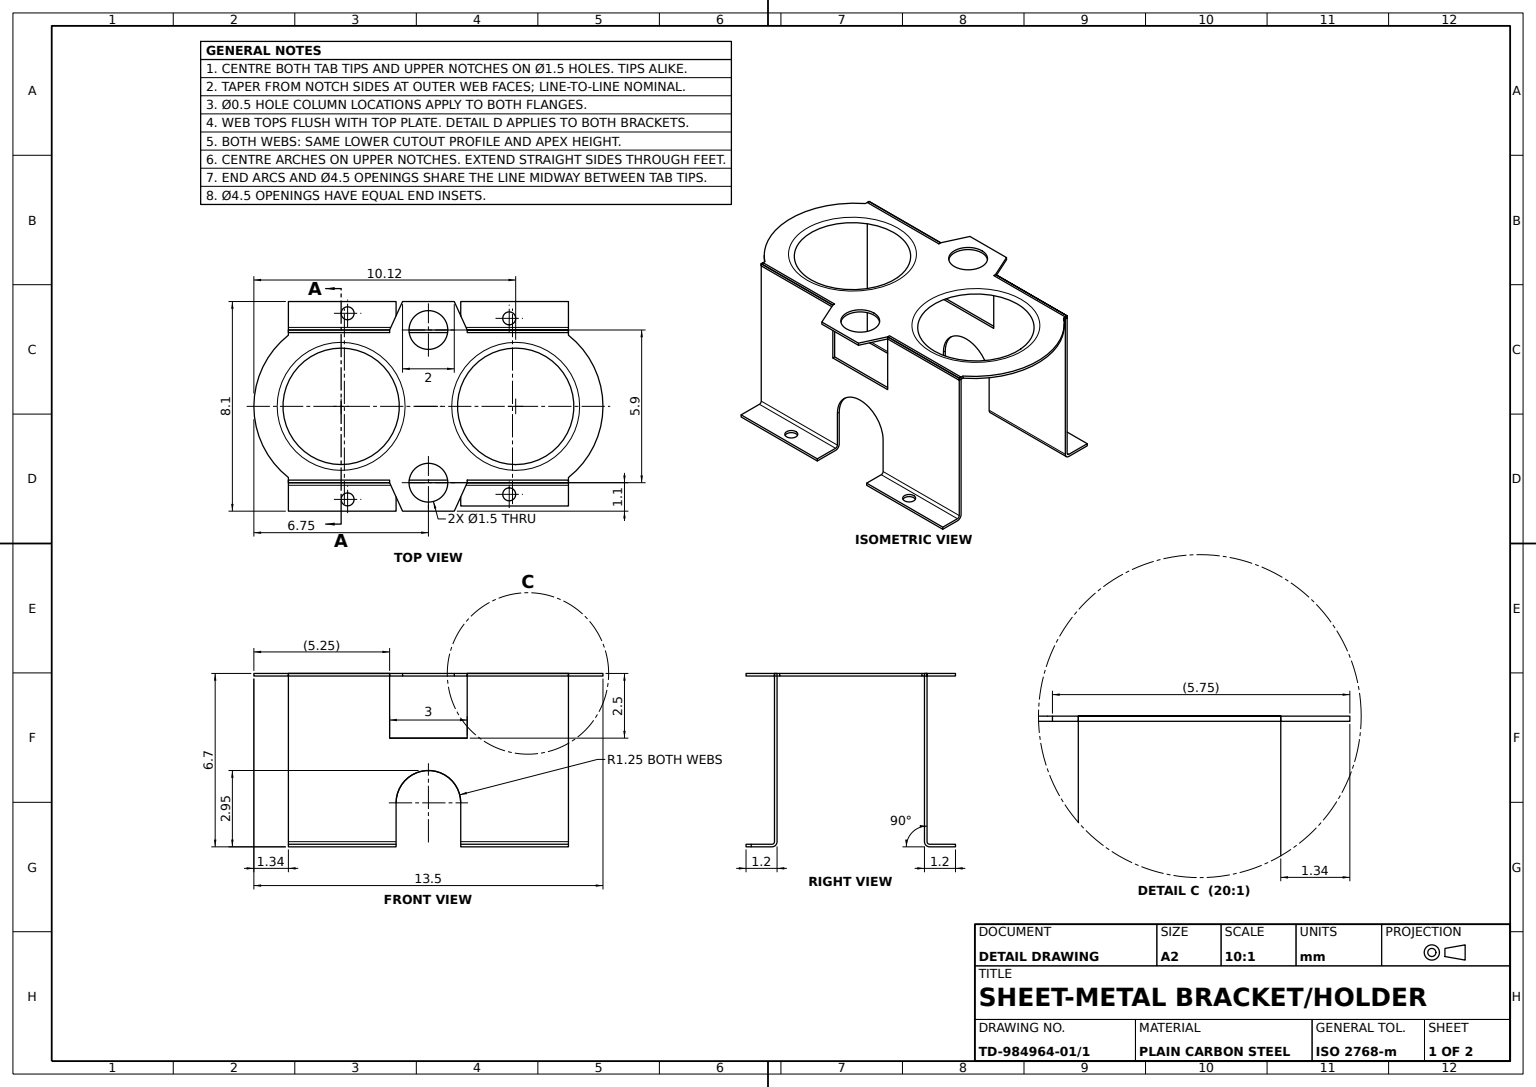
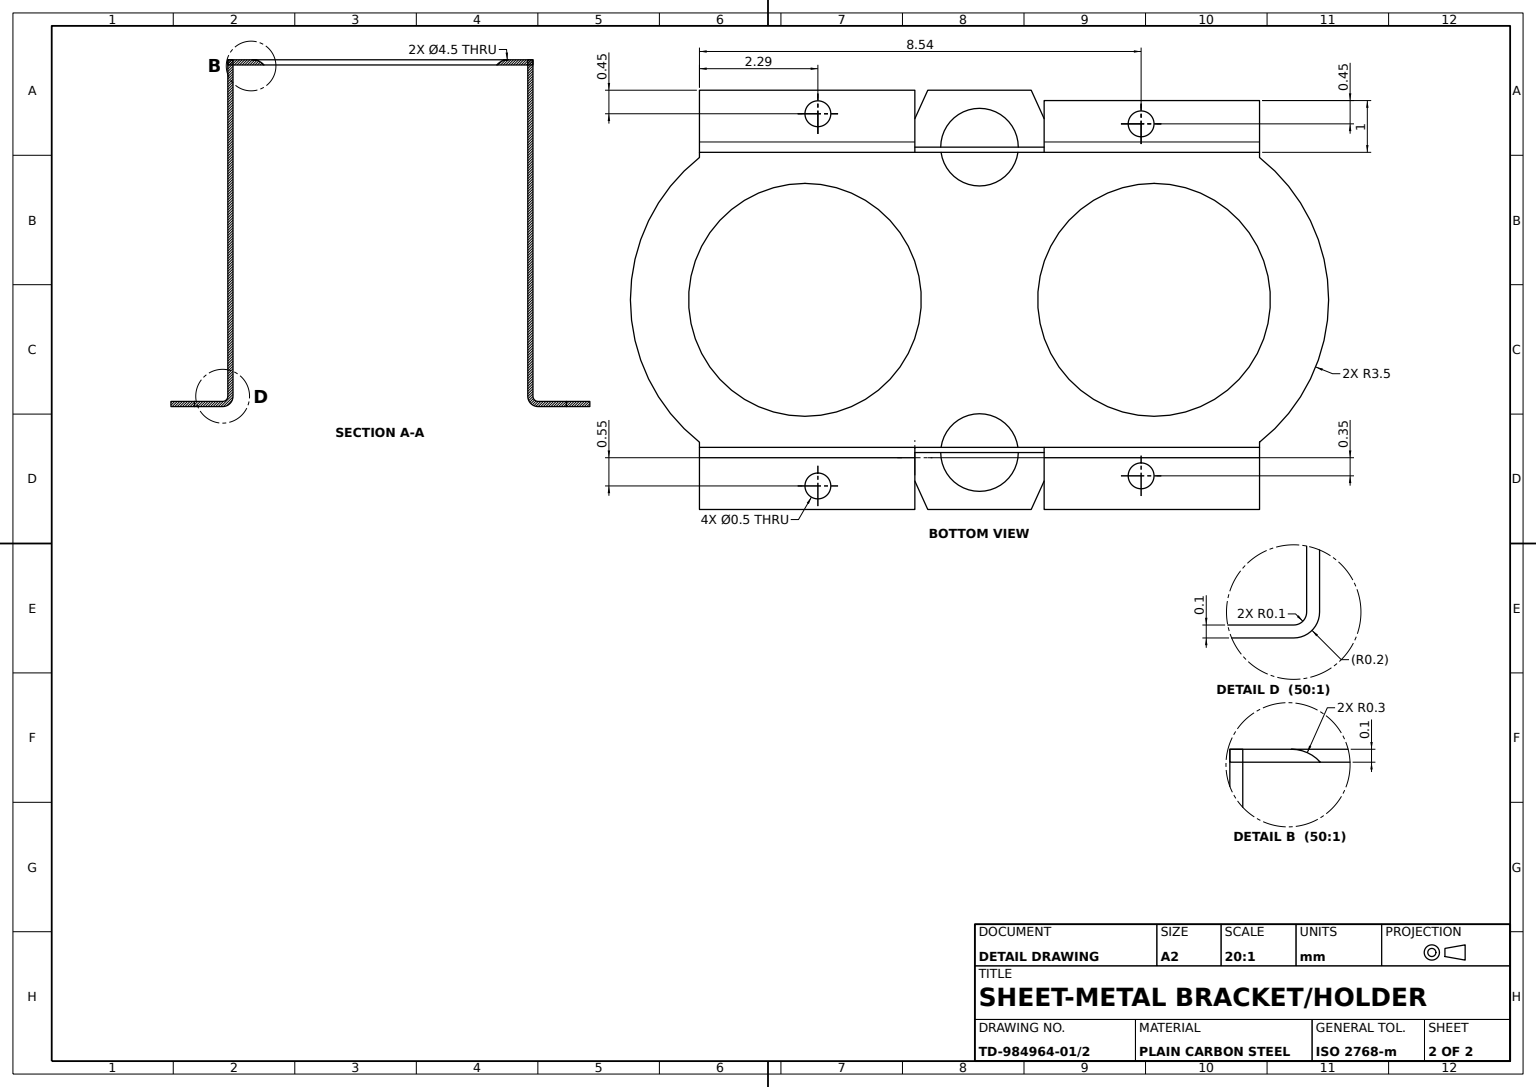
solid
v1 (3.375,0,-2.473607)
v2 (3.375,0,2.473607)
e1 v1 v2 CIRCLE(AX(P(3.375,0,0),D(0,-1,0),D(0,0,1)),2.473607)
v3 (3.375,-0.1,-2.25)
e2 v1 v3 CIRCLE(AX(P(3.375,-0.3,-2.473607),D(1,0,0),D(0,0,-1)),0.3)
v4 (3.375,-0.1,2.25)
e3 v4 v3 CIRCLE(AX(P(3.375,-0.1,0),D(0,1,0),D(0,0,-1)),2.25)
e4 v2 v4 CIRCLE(AX(P(3.375,-0.3,2.473607),D(-1,0,0),D(0,0,1)),0.3)
face TORUS(AX(P(3.375,-0.3,0),D(0,1,0),D(0,0,1)),2.473607,0.3) [-e1 e2 -e3 -e4]
v5 (-5.414993,0,-2.95)
v6 (-5.414993,0,-2.75)
e5 v5 v6 LINE
v7 (-5.414993,-0.1,-2.95)
e6 v7 v5 LINE
v8 (-5.414993,-0.1,-2.75)
e7 v7 v8 LINE
e8 v8 v6 LINE
face PLANE(AX(P(-5.414993,-0.1,-2.95),D(-1,0,0),D(0,0,1))) [-e5 -e6 e7 e8]
v9 (-1,0,4.05)
v10 (1,0,4.05)
e9 v9 v10 LINE
v11 (-1,-0.1,4.05)
e10 v11 v9 LINE
v12 (1,-0.1,4.05)
e11 v11 v12 LINE
e12 v12 v10 LINE
face PLANE(AX(P(-1,-0.1,4.05),D(0,0,1),D(1,0,0))) [-e9 -e10 e11 e12]
v13 (-1.5,-0.1,-2.95)
e13 v13 v7 LINE
v14 (-1.5,0,-2.95)
e14 v14 v5 LINE
e15 v13 v14 LINE
face PLANE(AX(P(-5.414993,-0.1,-2.95),D(0,0,-1),D(-1,0,0))) [e13 e6 -e14 -e15]
v15 (-1,-0.1,-4.05)
v16 (-1,0,-4.05)
e16 v15 v16 LINE
e17 v15 v13 LINE
e18 v16 v14 LINE
face PLANE(AX(P(-1,-0.1,-4.05),D(-0.910366477,0,-0.413802944),D(-0.413802944,0,0.910366477))) [-e16 e17 e15 -e18]
v17 (1.5,-0.1,2.95)
e19 v12 v17 LINE
v18 (1.5,0,2.95)
e20 v17 v18 LINE
e21 v10 v18 LINE
face PLANE(AX(P(1,-0.1,4.05),D(0.910366477,0,0.413802944),D(0.413802944,0,-0.910366477))) [-e12 e19 e20 -e21]
v19 (-3.375,0,2.473607)
v20 (-3.375,0,-2.473607)
e22 v19 v20 CIRCLE(AX(P(-3.375,0,0),D(0,-1,0),D(0,0,1)),2.473607)
v21 (-3.375,-0.1,2.25)
e23 v19 v21 CIRCLE(AX(P(-3.375,-0.3,2.473607),D(-1,0,0),D(0,0,1)),0.3)
v22 (-3.375,-0.1,-2.25)
e24 v22 v21 CIRCLE(AX(P(-3.375,-0.1,0),D(0,1,0),D(0,0,1)),2.25)
e25 v20 v22 CIRCLE(AX(P(-3.375,-0.3,-2.473607),D(1,0,0),D(0,0,-1)),0.3)
face TORUS(AX(P(-3.375,-0.3,0),D(0,1,0),D(0,0,1)),2.473607,0.3) [-e22 e23 -e24 -e25]
v23 (5.414993,0,2.95)
v24 (5.414993,0,2.75)
e26 v23 v24 LINE
v25 (5.414993,-0.1,2.95)
e27 v25 v23 LINE
v26 (5.414993,-0.1,2.75)
e28 v25 v26 LINE
e29 v26 v24 LINE
face PLANE(AX(P(5.414993,-0.1,2.95),D(1,0,0),D(0,0,-1))) [-e26 -e27 e28 e29]
e30 v17 v25 LINE
e31 v18 v23 LINE
face PLANE(AX(P(1.5,-0.1,2.95),D(0,0,1),D(1,0,0))) [-e20 e30 e27 -e31]
v27 (1,0,-4.05)
e32 v27 v16 LINE
v28 (1,-0.1,-4.05)
e33 v28 v27 LINE
e34 v28 v15 LINE
face PLANE(AX(P(-1,-0.1,-4.05),D(0,0,-1),D(-1,0,0))) [-e32 -e33 e34 e16]
v29 (5.414993,-0.1,-2.75)
v30 (5.414993,0,-2.75)
e35 v29 v30 LINE
e36 v24 v30 CIRCLE(AX(P(3.251947,0,0),D(0,1,0),D(0,0,1)),3.498753)
e37 v26 v29 CIRCLE(AX(P(3.251947,-0.1,0),D(0,1,0),D(0,0,1)),3.498753)
face CYL(AX(P(3.251947,-0.1,0),D(0,1,0),D(0,0,1)),3.498753) [e35 -e36 -e29 e37]
v31 (0,-0.1,3.7)
v32 (0,0,3.7)
e38 v31 v32 LINE
v33 (0,-0.1,2.2)
e39 v33 v31 CIRCLE(AX(P(0,-0.1,2.95),D(0,1,0),D(0,0,1)),0.75)
v34 (0,0,2.2)
e40 v33 v34 LINE
e41 v34 v32 CIRCLE(AX(P(0,0,2.95),D(0,1,0),D(0,0,1)),0.75)
face CYL(AX(P(0,-0.1,2.95),D(0,1,0),D(0,0,1)),0.75) rev [-e38 -e39 e40 e41]
v35 (-5.414993,-0.1,2.75)
e42 v8 v35 CIRCLE(AX(P(-3.250114,-0.1,0),D(0,1,0),D(0,0,-1)),3.499886)
v36 (-5.414993,0,2.75)
e43 v35 v36 LINE
e44 v6 v36 CIRCLE(AX(P(-3.250114,0,0),D(0,1,0),D(0,0,-1)),3.499886)
face CYL(AX(P(-3.250114,-0.1,0),D(0,1,0),D(0,0,1)),3.499886) [-e8 e42 e43 -e44]
v37 (5.414993,-0.1,-2.95)
e45 v29 v37 LINE
v38 (5.414993,0,-2.95)
e46 v37 v38 LINE
e47 v30 v38 LINE
face PLANE(AX(P(5.414993,-0.1,-2.95),D(1,0,0),D(0,0,-1))) [e45 e46 -e47 -e35]
v39 (0,-0.1,-3.7)
v40 (0,-0.1,-2.2)
e48 v39 v40 CIRCLE(AX(P(0,-0.1,-2.95),D(0,1,0),D(0,0,1)),0.75)
v41 (0,0,-3.7)
e49 v39 v41 LINE
v42 (0,0,-2.2)
e50 v41 v42 CIRCLE(AX(P(0,0,-2.95),D(0,1,0),D(0,0,1)),0.75)
e51 v40 v42 LINE
face CYL(AX(P(0,-0.1,-2.95),D(0,1,0),D(0,0,1)),0.75) rev [-e48 e49 e50 -e51]
e52 v40 v39 CIRCLE(AX(P(0,-0.1,-2.95),D(0,1,0),D(0,0,1)),0.75)
e53 v42 v41 CIRCLE(AX(P(0,0,-2.95),D(0,1,0),D(0,0,1)),0.75)
face CYL(AX(P(0,-0.1,-2.95),D(0,1,0),D(0,0,1)),0.75) rev [-e52 e51 e53 -e49]
v43 (-1.5,-0.1,2.95)
v44 (-1.5,0,2.95)
e54 v43 v44 LINE
e55 v43 v11 LINE
e56 v44 v9 LINE
face PLANE(AX(P(-1,-0.1,4.05),D(-0.910366477,0,0.413802944),D(0.413802944,0,0.910366477))) [-e54 e55 e10 -e56]
v45 (-5.414993,-0.1,2.95)
e57 v35 v45 LINE
v46 (-5.414993,0,2.95)
e58 v45 v46 LINE
e59 v36 v46 LINE
face PLANE(AX(P(-5.414993,-0.1,2.95),D(-1,0,0),D(0,0,1))) [-e43 e57 e58 -e59]
e60 v32 v34 CIRCLE(AX(P(0,0,2.95),D(0,1,0),D(0,0,1)),0.75)
e61 v31 v33 CIRCLE(AX(P(0,-0.1,2.95),D(0,1,0),D(0,0,1)),0.75)
face CYL(AX(P(0,-0.1,2.95),D(0,1,0),D(0,0,1)),0.75) rev [e38 e60 -e40 -e61]
e62 v21 v22 CIRCLE(AX(P(-3.375,-0.1,0),D(0,1,0),D(0,0,1)),2.25)
e63 v20 v19 CIRCLE(AX(P(-3.375,0,0),D(0,-1,0),D(0,0,1)),2.473607)
face TORUS(AX(P(-3.375,-0.3,0),D(0,1,0),D(0,0,1)),2.473607,0.3) [-e62 -e23 -e63 e25]
v47 (1.5,0,-2.95)
e64 v47 v27 LINE
v48 (1.5,-0.1,-2.95)
e65 v48 v47 LINE
e66 v48 v28 LINE
face PLANE(AX(P(1,-0.1,-4.05),D(0.910366477,0,-0.413802944),D(-0.413802944,0,-0.910366477))) [-e64 -e65 e66 e33]
e67 v38 v47 LINE
e68 v46 v44 LINE
e69 v2 v1 CIRCLE(AX(P(3.375,0,0),D(0,-1,0),D(0,0,1)),2.473607)
face PLANE(AX(P(3.251947,0,0),D(0,1,0),D(0,0,1))) [-e41 -e60] [e47 e67 e64 e32 e18 e14 e5 e44 e59 e68 e56 e9 e21 e31 e26 e36] [e22 e63] [e1 e69] [-e53 -e50]
e70 v37 v48 LINE
face PLANE(AX(P(1.5,-0.1,-2.95),D(0,0,-1),D(-1,0,0))) [-e67 -e46 e70 e65]
e71 v45 v43 LINE
face PLANE(AX(P(-5.414993,-0.1,2.95),D(0,0,1),D(1,0,0))) [e54 -e68 -e58 e71]
e72 v3 v4 CIRCLE(AX(P(3.375,-0.1,0),D(0,1,0),D(0,0,-1)),2.25)
face PLANE(AX(P(3.251947,-0.1,0),D(0,1,0),D(0,0,1))) rev [e39 e61] [e52 e48] [-e13 -e17 -e34 -e66 -e70 -e45 -e37 -e28 -e30 -e19 -e11 -e55 -e71 -e57 -e42 -e7] [e72 e3] [e62 e24]
face TORUS(AX(P(3.375,-0.3,0),D(0,1,0),D(0,0,1)),2.473607,0.3) [e4 -e72 -e2 -e69]
solid
v49 (-5.414993,-6.5,2.95)
v50 (-5.414993,-6.6,3.05)
e73 v49 v50 CIRCLE(AX(P(-5.414993,-6.5,3.05),D(-1,0,0),D(0,0,-1)),0.1)
v51 (-5.414993,-6.5,2.85)
e74 v51 v49 LINE
v52 (-5.414993,-6.7,3.05)
e75 v51 v52 CIRCLE(AX(P(-5.414993,-6.5,3.05),D(-1,0,0),D(0,0,-1)),0.2)
e76 v50 v52 LINE
face PLANE(AX(P(-5.414993,-6.5,3.05),D(-1,0,0),D(0,0,1))) [-e73 -e74 e75 -e76]
v53 (-1.25,-6.6,3.05)
e77 v50 v53 LINE
v54 (-5.414993,-6.6,4.05)
e78 v54 v50 LINE
v55 (-1.25,-6.6,4.05)
e79 v55 v54 LINE
e80 v53 v55 LINE
v56 (-3.125,-6.6,3.845112)
v57 (-3.125,-6.6,3.345112)
e81 v56 v57 CIRCLE(AX(P(-3.125,-6.6,3.595112),D(0,1,0),D(0,0,1)),0.25)
e82 v57 v56 CIRCLE(AX(P(-3.125,-6.6,3.595112),D(0,1,0),D(0,0,1)),0.25)
face PLANE(AX(P(0,-6.6,0),D(0,1,0),D(0,0,1))) [-e77 -e78 -e79 -e80] [-e81 -e82]
v58 (1.5,0,2.85)
v59 (1.5,-2.5,2.85)
e83 v58 v59 LINE
v60 (1.5,-2.5,2.95)
e84 v59 v60 LINE
v61 (1.5,0,2.95)
e85 v61 v60 LINE
e86 v58 v61 LINE
face PLANE(AX(P(1.5,-2.5,2.85),D(-1,0,0),D(0,0,1))) [e83 e84 -e85 -e86]
v62 (5.414993,-6.5,2.85)
v63 (5.414993,-6.5,2.95)
e87 v62 v63 LINE
v64 (5.414993,0,2.85)
e88 v62 v64 LINE
v65 (5.414993,0,2.95)
e89 v64 v65 LINE
e90 v63 v65 LINE
face PLANE(AX(P(5.414993,-6.5,2.85),D(1,0,0),D(0,0,-1))) [-e87 e88 e89 -e90]
e91 v64 v58 LINE
v66 (1.25,-6.5,2.85)
e92 v66 v62 LINE
v67 (1.25,-5,2.85)
e93 v67 v66 LINE
v68 (-1.25,-5,2.85)
e94 v68 v67 CIRCLE(AX(P(0,-5,2.85),D(0,0,-1),D(1,0,0)),1.25)
v69 (-1.25,-6.5,2.85)
e95 v69 v68 LINE
e96 v51 v69 LINE
v70 (-5.414993,0,2.85)
e97 v70 v51 LINE
v71 (-1.5,0,2.85)
e98 v71 v70 LINE
v72 (-1.5,-2.5,2.85)
e99 v72 v71 LINE
e100 v59 v72 LINE
face PLANE(AX(P(0,-5,2.85),D(0,0,1),D(1,0,0))) rev [-e83 -e91 -e88 -e92 -e93 -e94 -e95 -e96 -e97 -e98 -e99 -e100]
v73 (1.25,-6.7,3.85)
v74 (1.25,-6.6,3.85)
e101 v73 v74 LINE
v75 (5.414993,-6.7,3.85)
e102 v75 v73 LINE
v76 (5.414993,-6.6,3.85)
e103 v75 v76 LINE
e104 v76 v74 LINE
face PLANE(AX(P(1.25,-6.7,3.85),D(0,0,-1),D(0,1,0))) rev [-e101 -e102 e103 e104]
v77 (1.25,-5,2.95)
v78 (1.25,-6.5,2.95)
e105 v77 v78 LINE
e106 v67 v77 LINE
e107 v66 v78 LINE
face PLANE(AX(P(1.25,-5,2.85),D(-1,0,0),D(0,-1,0))) [-e105 -e106 e93 e107]
v79 (-1.5,-2.5,2.95)
e108 v72 v79 LINE
e109 v60 v79 LINE
face PLANE(AX(P(-1.5,-2.5,2.85),D(0,1,0),D(0,0,1))) [e108 -e109 -e84 e100]
v80 (-1.5,0,2.95)
v81 (-5.414993,0,2.95)
e110 v80 v81 LINE
e111 v71 v80 LINE
e112 v70 v81 LINE
face PLANE(AX(P(-1.5,0,2.85),D(0,1,0),D(-1,0,0))) [-e110 -e111 e98 e112]
v82 (-5.414993,-6.7,4.05)
e113 v82 v52 LINE
e114 v82 v54 LINE
face PLANE(AX(P(-5.414993,-6.7,2.95),D(1,0,0),D(0,1,0))) rev [e76 -e113 e114 e78]
v83 (-1.25,-6.5,2.95)
e115 v53 v83 CIRCLE(AX(P(-1.25,-6.5,3.05),D(1,0,0),D(0,0,-1)),0.1)
v84 (-1.25,-6.7,3.05)
e116 v53 v84 LINE
e117 v84 v69 CIRCLE(AX(P(-1.25,-6.5,3.05),D(1,0,0),D(0,0,-1)),0.2)
e118 v69 v83 LINE
face PLANE(AX(P(-1.25,-6.5,3.05),D(-1,0,0),D(0,0,1))) rev [-e115 e116 e117 e118]
v85 (-1.25,-5,2.95)
e119 v83 v85 LINE
e120 v85 v77 CIRCLE(AX(P(0,-5,2.95),D(0,0,-1),D(1,0,0)),1.25)
e121 v78 v63 LINE
e122 v65 v61 LINE
e123 v79 v80 LINE
e124 v81 v49 LINE
e125 v49 v83 LINE
face PLANE(AX(P(0,-5,2.95),D(0,0,1),D(1,0,0))) [e119 e120 e105 e121 e90 e122 e85 e109 e123 e110 e124 e125]
v86 (5.414993,-6.7,3.05)
e126 v86 v75 LINE
v87 (1.25,-6.7,3.05)
e127 v73 v87 LINE
e128 v86 v87 LINE
v88 (3.125,-6.7,3.65)
v89 (3.125,-6.7,3.15)
e129 v88 v89 CIRCLE(AX(P(3.125,-6.7,3.4),D(0,1,0),D(0,0,1)),0.25)
e130 v89 v88 CIRCLE(AX(P(3.125,-6.7,3.4),D(0,1,0),D(0,0,1)),0.25)
face PLANE(AX(P(0,-6.7,0),D(0,1,0),D(0,0,1))) rev [e126 e102 e127 -e128] [e129 e130]
v90 (-1.25,-6.7,4.05)
e131 v90 v55 LINE
e132 v84 v90 LINE
face PLANE(AX(P(-1.25,-6.7,4.05),D(-1,0,0),D(0,0,1))) rev [e80 -e131 -e132 -e116]
v91 (1.25,-6.6,3.05)
e133 v74 v91 LINE
e134 v91 v87 LINE
face PLANE(AX(P(1.25,-6.7,2.95),D(1,0,0),D(0,1,0))) rev [e133 e134 -e127 e101]
v92 (5.414993,-6.6,3.05)
e135 v92 v86 LINE
e136 v92 v76 LINE
face PLANE(AX(P(5.414993,-6.7,3.85),D(-1,0,0),D(0,0,1))) rev [-e135 e136 -e103 -e126]
e137 v92 v63 CIRCLE(AX(P(5.414993,-6.5,3.05),D(1,0,0),D(0,0,-1)),0.1)
e138 v86 v62 CIRCLE(AX(P(5.414993,-6.5,3.05),D(1,0,0),D(0,0,-1)),0.2)
face PLANE(AX(P(5.414993,-6.5,3.05),D(-1,0,0),D(0,0,1))) rev [e87 -e137 e135 e138]
face CYL(AX(P(-1.25,-6.5,3.05),D(1,0,0),D(0,-1,0)),0.1) rev [-e125 e73 e77 e115]
face PLANE(AX(P(-1.5,0,2.85),D(1,0,0),D(0,1,0))) [-e108 e99 e111 -e123]
e139 v68 v85 LINE
face CYL(AX(P(0,-5,2.85),D(0,0,1),D(1,0,0)),1.25) rev [-e139 e94 e106 -e120]
e140 v78 v91 CIRCLE(AX(P(1.25,-6.5,3.05),D(-1,0,0),D(0,0,-1)),0.1)
e141 v66 v87 CIRCLE(AX(P(1.25,-6.5,3.05),D(-1,0,0),D(0,0,-1)),0.2)
face PLANE(AX(P(1.25,-6.5,3.05),D(-1,0,0),D(0,0,1))) [-e134 -e140 -e107 e141]
face CYL(AX(P(5.414993,-6.5,3.05),D(1,0,0),D(0,-1,0)),0.2) [-e138 e128 -e141 e92]
face PLANE(AX(P(5.414993,0,2.85),D(0,1,0),D(-1,0,0))) [e91 e86 -e122 -e89]
v93 (3.125,-6.6,3.65)
e142 v93 v88 LINE
v94 (3.125,-6.6,3.15)
e143 v93 v94 CIRCLE(AX(P(3.125,-6.6,3.4),D(0,1,0),D(0,0,1)),0.25)
e144 v94 v89 LINE
face CYL(AX(P(3.125,-6.2,3.4),D(0,-1,0),D(0,0,-1)),0.25) rev [-e142 e143 e144 -e129]
v95 (-3.125,-6.7,3.845112)
e145 v56 v95 LINE
v96 (-3.125,-6.7,3.345112)
e146 v96 v95 CIRCLE(AX(P(-3.125,-6.7,3.595112),D(0,1,0),D(0,0,1)),0.25)
e147 v57 v96 LINE
face CYL(AX(P(-3.125,-6.2,3.595112),D(0,-1,0),D(0,0,-1)),0.25) rev [e82 e145 -e146 -e147]
e148 v84 v52 LINE
e149 v90 v82 LINE
e150 v95 v96 CIRCLE(AX(P(-3.125,-6.7,3.595112),D(0,1,0),D(0,0,1)),0.25)
face PLANE(AX(P(0,-6.7,0),D(0,1,0),D(0,0,1))) rev [e113 -e148 e132 e149] [e150 e146]
face CYL(AX(P(-3.125,-6.2,3.595112),D(0,-1,0),D(0,0,-1)),0.25) rev [-e150 -e145 e81 e147]
e151 v94 v93 CIRCLE(AX(P(3.125,-6.6,3.4),D(0,1,0),D(0,0,1)),0.25)
e152 v91 v92 LINE
face PLANE(AX(P(0,-6.6,0),D(0,1,0),D(0,0,1))) [-e151 -e143] [-e152 -e133 -e104 -e136]
face PLANE(AX(P(-5.414993,-6.7,4.05),D(0,0,-1),D(0,1,0))) rev [e131 e79 -e114 -e149]
face CYL(AX(P(-1.25,-6.5,3.05),D(1,0,0),D(0,-1,0)),0.2) [e96 -e117 e148 -e75]
face CYL(AX(P(3.125,-6.2,3.4),D(0,-1,0),D(0,0,-1)),0.25) rev [e142 -e130 -e144 e151]
face PLANE(AX(P(-5.414993,-6.5,2.85),D(-1,0,0),D(0,0,1))) [e74 -e124 -e112 e97]
face CYL(AX(P(5.414993,-6.5,3.05),D(1,0,0),D(0,-1,0)),0.1) rev [-e121 e140 e152 e137]
face PLANE(AX(P(-1.25,-5,2.85),D(1,0,0),D(0,1,0))) [-e119 -e118 e95 e139]
solid
v97 (1.25,-6.7,-4.05)
v98 (1.25,-6.6,-4.05)
e153 v97 v98 LINE
v99 (1.25,-6.7,-3.05)
e154 v99 v97 LINE
v100 (1.25,-6.6,-3.05)
e155 v100 v99 LINE
e156 v100 v98 LINE
face PLANE(AX(P(1.25,-6.7,-4.05),D(1,0,0),D(0,0,-1))) rev [-e153 -e154 -e155 e156]
v101 (3.125,-6.6,-3.65)
v102 (3.125,-6.7,-3.65)
e157 v101 v102 LINE
v103 (3.125,-6.6,-3.15)
e158 v103 v101 CIRCLE(AX(P(3.125,-6.6,-3.4),D(0,-1,0),D(0,0,1)),0.25)
v104 (3.125,-6.7,-3.15)
e159 v103 v104 LINE
e160 v104 v102 CIRCLE(AX(P(3.125,-6.7,-3.4),D(0,-1,0),D(0,0,1)),0.25)
face CYL(AX(P(3.125,-6.2,-3.4),D(0,-1,0),D(0,0,-1)),0.25) rev [-e157 -e158 e159 e160]
v105 (5.414993,-6.7,-4.05)
e161 v97 v105 LINE
v106 (5.414993,-6.6,-4.05)
e162 v98 v106 LINE
e163 v105 v106 LINE
face PLANE(AX(P(5.414993,-6.7,-4.05),D(0,0,1),D(0,-1,0))) rev [-e161 e153 e162 -e163]
v107 (1.5,0,-2.85)
v108 (1.5,0,-2.95)
e164 v107 v108 LINE
v109 (1.5,-2.5,-2.95)
e165 v108 v109 LINE
v110 (1.5,-2.5,-2.85)
e166 v110 v109 LINE
e167 v107 v110 LINE
face PLANE(AX(P(1.5,0,-2.85),D(1,0,0),D(0,0,-1))) rev [e164 e165 -e166 -e167]
e168 v101 v103 CIRCLE(AX(P(3.125,-6.6,-3.4),D(0,-1,0),D(0,0,1)),0.25)
e169 v102 v104 CIRCLE(AX(P(3.125,-6.7,-3.4),D(0,-1,0),D(0,0,1)),0.25)
face CYL(AX(P(3.125,-6.2,-3.4),D(0,-1,0),D(0,0,-1)),0.25) rev [-e159 -e168 e157 e169]
v111 (-5.414993,-6.6,-4.05)
v112 (-1.25,-6.6,-4.05)
e170 v111 v112 LINE
v113 (-5.414993,-6.6,-3.05)
e171 v113 v111 LINE
v114 (-1.25,-6.6,-3.05)
e172 v114 v113 LINE
e173 v112 v114 LINE
v115 (-3.125,-6.6,-3.345112)
v116 (-3.125,-6.6,-3.845112)
e174 v115 v116 CIRCLE(AX(P(-3.125,-6.6,-3.595112),D(0,-1,0),D(0,0,1)),0.25)
e175 v116 v115 CIRCLE(AX(P(-3.125,-6.6,-3.595112),D(0,-1,0),D(0,0,1)),0.25)
face PLANE(AX(P(0,-6.6,0),D(0,1,0),D(0,0,1))) [-e170 -e171 -e172 -e173] [e174 e175]
v117 (1.25,-5,-2.85)
v118 (1.25,-5,-2.95)
e176 v117 v118 LINE
v119 (-1.25,-5,-2.85)
e177 v119 v117 CIRCLE(AX(P(0,-5,-2.85),D(0,0,-1),D(1,0,0)),1.25)
v120 (-1.25,-5,-2.95)
e178 v119 v120 LINE
e179 v120 v118 CIRCLE(AX(P(0,-5,-2.95),D(0,0,-1),D(1,0,0)),1.25)
face CYL(AX(P(0,-5,-2.85),D(0,0,-1),D(-1,0,0)),1.25) rev [-e176 -e177 e178 e179]
v121 (5.414993,-6.5,-2.85)
v122 (5.414993,-6.5,-2.95)
e180 v121 v122 LINE
v123 (5.414993,0,-2.95)
e181 v122 v123 LINE
v124 (5.414993,0,-2.85)
e182 v124 v123 LINE
e183 v121 v124 LINE
face PLANE(AX(P(5.414993,-6.5,-2.85),D(-1,0,0),D(0,0,1))) rev [e180 e181 -e182 -e183]
v125 (-5.414993,-6.5,-2.95)
e184 v113 v125 CIRCLE(AX(P(-5.414993,-6.5,-3.05),D(-1,0,0),D(0,0,1)),0.1)
v126 (-5.414993,-6.7,-3.05)
e185 v113 v126 LINE
v127 (-5.414993,-6.5,-2.85)
e186 v126 v127 CIRCLE(AX(P(-5.414993,-6.5,-3.05),D(-1,0,0),D(0,0,1)),0.2)
e187 v127 v125 LINE
face PLANE(AX(P(-5.414993,-6.5,-3.05),D(1,0,0),D(0,0,-1))) rev [-e184 e185 e186 e187]
v128 (-5.414993,-6.7,-4.05)
e188 v128 v111 LINE
e189 v126 v128 LINE
face PLANE(AX(P(-5.414993,-6.7,-4.05),D(1,0,0),D(0,0,-1))) rev [-e188 -e189 -e185 e171]
v129 (1.25,-6.5,-2.85)
e190 v117 v129 LINE
v130 (1.25,-6.5,-2.95)
e191 v118 v130 LINE
e192 v129 v130 LINE
face PLANE(AX(P(1.25,-5,-2.85),D(1,0,0),D(0,1,0))) rev [-e190 e176 e191 -e192]
v131 (-3.125,-6.7,-3.845112)
v132 (-3.125,-6.7,-3.345112)
e193 v131 v132 CIRCLE(AX(P(-3.125,-6.7,-3.595112),D(0,-1,0),D(0,0,1)),0.25)
e194 v132 v131 CIRCLE(AX(P(-3.125,-6.7,-3.595112),D(0,-1,0),D(0,0,1)),0.25)
v133 (-1.25,-6.7,-4.05)
e195 v128 v133 LINE
v134 (-1.25,-6.7,-3.05)
e196 v133 v134 LINE
e197 v126 v134 LINE
face PLANE(AX(P(0,-6.7,0),D(0,1,0),D(0,0,1))) rev [-e193 -e194] [e189 e195 e196 -e197]
e198 v123 v108 LINE
e199 v124 v107 LINE
face PLANE(AX(P(1.5,0,-2.85),D(0,-1,0),D(1,0,0))) rev [e198 -e164 -e199 e182]
e200 v100 v130 CIRCLE(AX(P(1.25,-6.5,-3.05),D(-1,0,0),D(0,0,1)),0.1)
e201 v99 v129 CIRCLE(AX(P(1.25,-6.5,-3.05),D(-1,0,0),D(0,0,1)),0.2)
face PLANE(AX(P(1.25,-6.5,-3.05),D(1,0,0),D(0,0,-1))) rev [-e200 e155 e201 e192]
v135 (-1.5,0,-2.95)
v136 (-5.414993,0,-2.95)
e202 v135 v136 LINE
v137 (-1.5,-2.5,-2.95)
e203 v137 v135 LINE
e204 v109 v137 LINE
e205 v130 v122 LINE
v138 (-1.25,-6.5,-2.95)
e206 v138 v120 LINE
e207 v125 v138 LINE
e208 v136 v125 LINE
face PLANE(AX(P(0,-5,-2.95),D(0,0,1),D(1,0,0))) rev [-e202 -e203 -e204 -e165 -e198 -e181 -e205 -e191 -e179 -e206 -e207 -e208]
e209 v133 v112 LINE
face PLANE(AX(P(-1.25,-6.7,-4.05),D(0,0,1),D(0,-1,0))) rev [e170 -e209 -e195 e188]
v139 (5.414993,-6.6,-3.05)
e210 v122 v139 CIRCLE(AX(P(5.414993,-6.5,-3.05),D(1,0,0),D(0,0,1)),0.1)
e211 v139 v100 LINE
face CYL(AX(P(1.25,-6.5,-3.05),D(-1,0,0),D(0,-1,0)),0.1) rev [e210 e211 e200 e205]
v140 (5.414993,-6.7,-3.05)
e212 v99 v140 LINE
e213 v121 v140 CIRCLE(AX(P(5.414993,-6.5,-3.05),D(1,0,0),D(0,0,1)),0.2)
e214 v129 v121 LINE
face CYL(AX(P(1.25,-6.5,-3.05),D(-1,0,0),D(0,-1,0)),0.2) [e212 -e213 -e214 -e201]
v141 (-1.25,-6.5,-2.85)
e215 v141 v134 CIRCLE(AX(P(-1.25,-6.5,-3.05),D(1,0,0),D(0,0,1)),0.2)
e216 v127 v141 LINE
face CYL(AX(P(-5.414993,-6.5,-3.05),D(-1,0,0),D(0,-1,0)),0.2) [-e215 -e216 -e186 e197]
e217 v116 v131 LINE
e218 v115 v132 LINE
face CYL(AX(P(-3.125,-6.2,-3.595112),D(0,-1,0),D(0,0,-1)),0.25) rev [-e175 e217 e193 -e218]
e219 v138 v114 CIRCLE(AX(P(-1.25,-6.5,-3.05),D(1,0,0),D(0,0,1)),0.1)
face CYL(AX(P(-5.414993,-6.5,-3.05),D(-1,0,0),D(0,-1,0)),0.1) rev [e219 e172 e184 e207]
face CYL(AX(P(-3.125,-6.2,-3.595112),D(0,-1,0),D(0,0,-1)),0.25) rev [-e174 e218 e194 -e217]
v142 (-1.5,-2.5,-2.85)
e220 v110 v142 LINE
v143 (-1.5,0,-2.85)
e221 v142 v143 LINE
v144 (-5.414993,0,-2.85)
e222 v143 v144 LINE
e223 v144 v127 LINE
e224 v141 v119 LINE
face PLANE(AX(P(0,-5,-2.85),D(0,0,1),D(1,0,0))) [e177 e190 e214 e183 e199 e167 e220 e221 e222 e223 e216 e224]
e225 v106 v139 LINE
face PLANE(AX(P(0,-6.6,0),D(0,1,0),D(0,0,1))) [-e211 -e225 -e162 -e156] [e158 e168]
e226 v143 v135 LINE
e227 v142 v137 LINE
face PLANE(AX(P(-1.5,-2.5,-2.85),D(-1,0,0),D(0,-1,0))) rev [e203 -e226 -e221 e227]
e228 v139 v140 LINE
face PLANE(AX(P(5.414993,-6.5,-3.05),D(1,0,0),D(0,0,-1))) [e213 -e228 -e210 -e180]
e229 v144 v136 LINE
face PLANE(AX(P(-5.414993,0,-2.85),D(1,0,0),D(0,0,-1))) rev [-e223 e229 e208 -e187]
e230 v141 v138 LINE
e231 v114 v134 LINE
face PLANE(AX(P(-1.25,-6.5,-3.05),D(1,0,0),D(0,0,-1))) [-e230 e215 -e231 -e219]
e232 v105 v140 LINE
face PLANE(AX(P(5.414993,-6.7,-2.95),D(-1,0,0),D(0,-1,0))) rev [e228 -e232 e163 e225]
face PLANE(AX(P(-1.25,-6.7,-2.95),D(-1,0,0),D(0,-1,0))) rev [-e196 e209 e173 e231]
face PLANE(AX(P(1.5,-2.5,-2.85),D(0,-1,0),D(0,0,-1))) rev [e166 e204 -e227 -e220]
face PLANE(AX(P(-5.414993,0,-2.85),D(0,-1,0),D(1,0,0))) rev [-e222 e226 e202 -e229]
face PLANE(AX(P(-1.25,-6.5,-2.85),D(-1,0,0),D(0,-1,0))) rev [-e178 -e224 e230 e206]
face PLANE(AX(P(0,-6.7,0),D(0,1,0),D(0,0,1))) rev [-e212 e154 e161 e232] [-e169 -e160]
